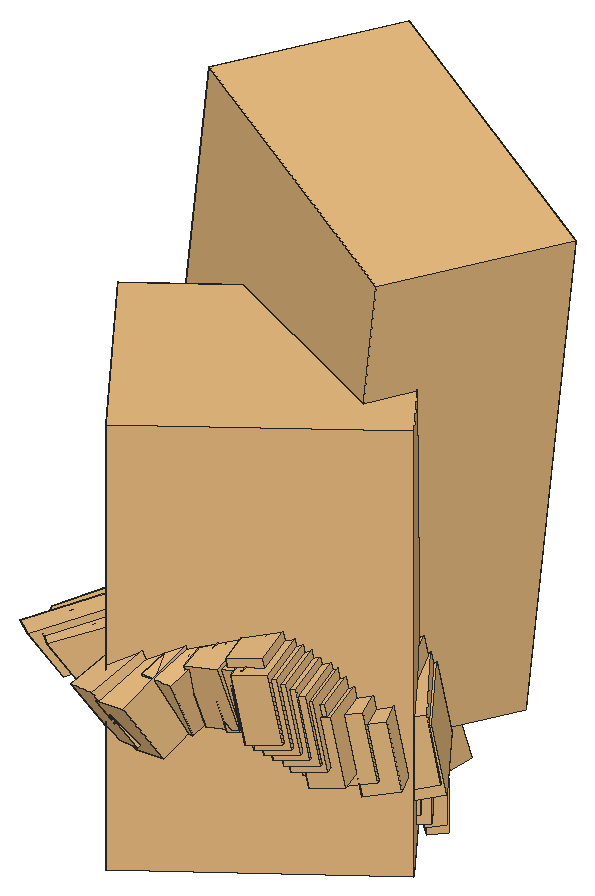
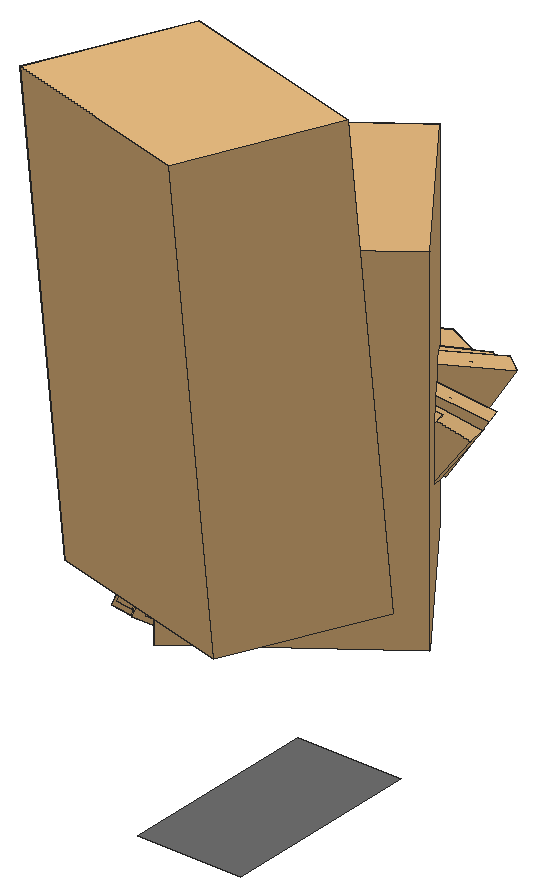
# SketchUp Ruby script. Lengths in inches.
U = 1.inch
M = Sketchup.active_model
def pt(a) = Geom::Point3d.new(a.map { |v| v * U })
def face(e, loops, mat)
  f = e.add_face(loops[0].map { |a| pt(a) })
  loops[1..].each { |l| e.add_face(l.map { |a| pt(a) }).erase! }
  f.material = f.back_material = mat if mat
  f
end
# faces: each face lists its corners as indices into pts; further lists are holes
def faces(e, pts, list, mat = nil) = list.each { |f| face(e, (f[0].is_a?(Array) ? f : [f]).map { |l| l.map { |i| pts[i] } }, mat) }
# xy, xz, yz: faces in a plane at the given z, y or x. An outline is a flat list of corners, or four numbers for a rectangle; further outlines are holes
def ring(l) = l.size == 4 ? [[l[0], l[1]], [l[2], l[1]], [l[2], l[3]], [l[0], l[3]]] : l.each_slice(2).to_a
def flat(e, list, mat, &to3) = list.each { |f| face(e, (f[0].is_a?(Array) ? f : [f]).map { |l| ring(l).map { |u, v| to3.(u, v) } }, mat) }
def xy(e, z, list, mat = nil) = flat(e, list, mat) { |x, y| [x, y, z] }
def xz(e, y, list, mat = nil) = flat(e, list, mat) { |x, z| [x, y, z] }
def yz(e, x, list, mat = nil) = flat(e, list, mat) { |y, z| [x, y, z] }
def lines(e, pts, list) = list.each { |a, b| e.add_line(pt(pts[a]), pt(pts[b])) }
# prism: a flat outline (further loops are holes) pulled along v
def prism(e, loops, v, mat = nil)
  f = face(e, loops, mat); d = Geom::Vector3d.new(v.map { |x| x * U })
  f.pushpull(f.normal.samedirection?(d) ? d.length : -d.length)
end
def box(e, o, s, mat = nil) = prism(e, [[o, [o[0] + s[0], o[1], o[2]], [o[0] + s[0], o[1] + s[1], o[2]], [o[0], o[1] + s[1], o[2]]]], [0, 0, s[2]], mat)
def at(x, y, z, deg = 0) = Geom::Transformation.translation(pt([x, y, z])) * Geom::Transformation.rotation(ORIGIN, Z_AXIS, deg.degrees)
def axes(o, x, y, z) = Geom::Transformation.new([*x, 0, *y, 0, *z, 0, *pt(o).to_a, 1])
def part(name) = M.definitions.add(name)
# library, detail: a bought-in or finely detailed component or shape, given as its bounding box
def library(name, o, s) = part(name).tap { |d| box(d.entities, o, s) }
def detail(e, o, s) = box(e.add_group.entities, o, s)
def put(e, d, t, mat = nil) = e.add_instance(d, t).tap { |i| i.material = mat if mat }
def group(e, t, mat = nil) = e.add_group.tap { |g| g.transformation = t; g.material = mat if mat }.entities
root = M.entities
M.materials.add("AM85_043_stem").color = [137, 75, 57]
M.materials.add("Generic\#4").color = [113, 113, 113]
c1 = library("Group\#263",[26.16,5.88,-22.96],[170.57,196.24,312.95])
c2 = part("Leaf blade")
p = [[83.87,1.9,45.32],[93.74,4.15,37.73],[37.05,-3.5625,61.7],[49.38,-2.58,60.05],[69.4,9.27,54.68],[74.7,9.96,52.16],
  [102.49,6.87,29.18],[110.02,10.09,19.93],[45.83,5.6,61.35],[51.45,6.53,60.35],[91.18,12.19,41.53],[94.56,12.64,38.66],
  [12.82,-5.2,59.53],[24.77,-4.41,61.53],[22.59,0.63,61.46],[34.04,3.3,62.19],[61.47,-1.4,56.68],[73.04,0.08,51.71],
  [109.02,14.97,22.84],[115.89,16.47,11.9375]]
lines(c2.entities,p,[[0,1],[2,3],[4,5],[6,7],[8,9],[10,11],[12,13],[14,15],[16,17],[18,19]])
detail(c2.entities,[1.52,-6.02,0.37],[119.64,24.16,61.82])
c3 = part("Group\#250")
p = [[69.397,177.044,-76.908],[69.056,177.22,-76.772],[69.397,177.397,-76.635],[69.739,177.22,-76.772],[69.397,126.923,-36.489],[68.124,127.405,-35.832],
  [69.397,153.661,-55.129],[70.671,127.405,-35.832],[68.59,154.026,-54.756],[70.205,154.026,-54.756],[69.397,127.887,-35.175],[69.397,154.392,-54.384],
  [69.397,97.5,-21.509],[67.658,98.015,-20.533],[71.137,98.015,-20.533],[69.397,98.53,-19.558],[69.397,66.147,-10.6],[67.192,66.605,-9.289],
  [71.603,66.605,-9.289],[69.397,67.064,-7.977],[69.397,33.682,-4.048],[66.726,33.994,-2.4],[72.069,33.994,-2.4],[69.397,34.304,-0.752],
  [69.397,0.958,-2],[66.26,1.035,-0.035],[69.397,1.112,1.931],[72.535,1.035,-0.035],[69.397,0.956,-2]]
faces(c3.entities,p,[[0,1,2,3]])
faces(c3.entities,p,[[4,5,6],[4,6,7],[8,6,5],[9,7,6],[5,10,11,8],[7,9,11,10],[12,13,4],[12,4,14],
  [5,4,13],[7,14,4],[13,15,10,5],[14,7,10,15],[16,17,12],[16,12,18],[13,12,17],[14,18,12],
  [17,19,15,13],[18,14,15,19],[16,20,17],[16,18,20],[21,17,20],[22,20,18],[21,23,17],[22,18,23],
  [19,17,23],[19,23,18],[20,24,21],[20,22,24],[25,21,24],[25,26,21],[27,24,22],[22,23,27],
  [23,21,26],[28,25,24],[28,27,25],[28,24,27],[26,27,23],[26,25,27]],"AM85_043_stem")
c4 = library("Group\#270",[27.32,5.88,-22.96],[171.91,196.24,312.95])
xy(root,62.5,[[443.58,67.75,455.52,90.9375]],"Generic\#4")
put(root,c1,axes([470.25,54.41,79.57],[0.04473,0.09619,-0.00136],[-0.14118,0.06602,0.02589],[0.02371,-0.00888,0.15193]))
g1 = group(root,at(474.43,72.34,71.32))
put(g1,c2,axes([-12.11,-1.61,3.27],[0.03868,-0.0392,0.03775],[-0.05285,-0.06013,-0.01977],[-0.04833,0.01698,0.0709]))
put(g1,c2,axes([-11.96,-0.56,4.01],[0.04263,-0.04823,0.03034],[-0.05668,-0.05579,-0.02374],[-0.0425,0.00994,0.07598]))
put(g1,c2,axes([-9.03,-15.24,6.15],[0.03132,0.06406,0.00852],[-0.06704,0.0181,-0.03972],[-0.0425,0.00994,0.07598]))
put(g1,c2,axes([-0.71,-1.03,-0.15],[0.01778,-0.047,0.01638],[-0.07034,-0.03079,-0.03479],[-0.0425,0.00994,0.07598]))
put(g1,c2,axes([-18.94,-8.86,3.45],[0.06742,0.02078,0.03933],[0.01295,-0.07484,0.01772],[-0.04843,0.00252,0.04485]))
put(g1,c2,axes([-7.92,0.23,1.4375],[0.0479,-0.05419,0.03409],[-0.05668,-0.05579,-0.02374],[-0.0425,0.00994,0.07598]))
put(g1,c2,axes([-4.09,0.28,0.43],[0.03378,-0.05538,0.02642],[-0.06587,-0.03995,-0.03103],[-0.0425,0.00994,0.07598]))
put(g1,c2,axes([-1.25,-0.99,0.48],[0.01778,-0.047,0.01638],[-0.07034,-0.03079,-0.03479],[-0.0425,0.00994,0.07598]))
put(g1,c2,axes([-7.45,0.48,0.7],[0.0479,-0.05419,0.03409],[-0.05668,-0.05579,-0.02374],[-0.0425,0.00994,0.07598]))
put(g1,c2,axes([-10.4,-14,5.8125],[0.02588,0.05213,0.018],[-0.0646,0.02369,-0.03789],[-0.04616,0.00147,0.07425]))
put(g1,c2,axes([-12.98,-2.44,3.14],[0.0395,-0.03313,0.03981],[-0.04826,-0.06412,-0.01628],[-0.05052,0.01802,0.06901]))
put(g1,c2,axes([-8.82,0.5,1.72],[0.0479,-0.05419,0.03409],[-0.05668,-0.05579,-0.02374],[-0.0425,0.00994,0.07598]))
put(g1,c2,axes([-15.65,-13.52,2.6],[0.04629,0.04424,0.05183],[-0.03259,0.05072,-0.03419],[-0.06385,0.00038,0.05972]))
put(g1,c2,axes([-14.34,-14.04,2.61],[0.03849,0.04933,0.05152],[-0.04598,0.04493,-0.0315],[-0.06071,-0.00886,0.06145]))
put(g1,c2,axes([-6.64,-15.3,5],[0.03132,0.06406,0.00852],[-0.06704,0.0181,-0.03972],[-0.0425,0.00994,0.07598]))
put(g1,c2,axes([-6.11,-15.16,5.27],[0.03132,0.06406,0.00852],[-0.06704,0.0181,-0.03972],[-0.0425,0.00994,0.07598]))
put(g1,c2,axes([-7.43,-15.45,5.63],[0.03132,0.06406,0.00852],[-0.06704,0.0181,-0.03972],[-0.0425,0.00994,0.07598]))
put(g1,c2,axes([-9.33,0.5,2.05],[0.0479,-0.05419,0.03409],[-0.05668,-0.05579,-0.02374],[-0.0425,0.00994,0.07598]))
put(g1,c2,axes([-15.7,-4.11,0.6],[0.04795,-0.01809,0.0661],[-0.02929,-0.07414,-0.00575],[-0.06447,0.01799,0.05565]))
put(g1,c2,axes([-18.72,-10.18,4.28],[0.06811,0.01591,0.04038],[-0.00659,0.06451,-0.01242],[-0.04843,0.00252,0.04485]))
put(g1,c2,axes([-2.05,-14.43,3.48],[0.0178,0.05862,0.00176],[-0.07169,0.00154,-0.04001],[-0.0425,0.00994,0.07598]))
put(g1,c2,axes([0.37,-12.77,2.89],[0.00491,0.04484,-0.00348],[-0.07359,-0.00764,-0.03979],[-0.0425,0.00994,0.07598]))
put(g1,c2,axes([-5.26,-15.32,3.98],[0.03132,0.06406,0.00852],[-0.06704,0.0181,-0.03972],[-0.0425,0.00994,0.07598]))
put(g1,c2,axes([-9.62,-14.86,6.93],[0.02788,0.05702,0.00758],[-0.06704,0.0181,-0.03972],[-0.0425,0.00994,0.07598]))
put(g1,c2,axes([-8.5,-15.29,5.87],[0.03132,0.06406,0.00852],[-0.06704,0.0181,-0.03972],[-0.0425,0.00994,0.07598]))
put(g1,c2,axes([-10.56,0.27,2.66],[0.0479,-0.05419,0.03409],[-0.05668,-0.05579,-0.02374],[-0.0425,0.00994,0.07598]))
put(g1,c2,axes([-11.77,0.21,3.21],[0.0479,-0.05419,0.03409],[-0.05668,-0.05579,-0.02374],[-0.0425,0.00994,0.07598]))
put(g1,c2,axes([-16.81,-5.04,0.9],[0.05394,-0.01033,0.06364],[-0.01462,-0.07744,-0.00647],[-0.06473,0.00665,0.05837]))
put(g1,c2,axes([-11.17,0.24,2.9375],[0.0479,-0.05419,0.03409],[-0.05668,-0.05579,-0.02374],[-0.0425,0.00994,0.07598]))
put(g1,c2,axes([-9.95,0.3,2.38],[0.0479,-0.05419,0.03409],[-0.05668,-0.05579,-0.02374],[-0.0425,0.00994,0.07598]))
put(g1,c2,axes([-9.77,-14.44,6.8],[0.02788,0.05702,0.00758],[-0.06704,0.0181,-0.03972],[-0.0425,0.00994,0.07598]))
put(g1,c2,axes([-14.52,-4.3,2.14],[0.04432,-0.01726,0.05016],[-0.04066,-0.06954,0.00497],[-0.053,0.02967,0.06181]))
put(g1,c2,axes([-11.4375,-13.65,5.43],[0.02804,0.04864,0.02213],[-0.06132,0.02903,-0.03642],[-0.04792,-0.00053,0.07303]))
put(g1,c2,axes([-5.5,0.05,0.88],[0.03829,-0.05246,0.02852],[-0.06335,-0.04371,-0.02912],[-0.0425,0.00994,0.07598]))
put(g1,c2,axes([-8.12,-15.34,6.33],[0.03132,0.06406,0.00852],[-0.06704,0.0181,-0.03972],[-0.0425,0.00994,0.07598]))
put(g1,c2,axes([-13.32,-13.04,3.89],[0.03602,0.042,0.03735],[-0.05638,0.04265,-0.0193],[-0.04711,-0.0123,0.07089]))
put(g1,c2,axes([-3.5,-14.44,3.88],[0.02275,0.05837,0.00455],[-0.07027,0.00563,-0.03979],[-0.0425,0.00994,0.07598]))
put(g1,c3,axes([-0.41,-1.05,-0.14],[0.01308,-0.09333,0.02018],[-0.04855,0.00674,0.06494],[0.06476,0.01996,0.05057]))
put(root,c4,axes([484.52,51.8,73.52],[-0.0818,0.11119,0],[-0.10263,-0.0755,0],[0,0,0.13246]))
g2 = group(root,at(483.76,57.21,77.5))
put(g2,c2,axes([-10.8,-12.78,7.47],[-0.02264,0.10412,0.02015],[-0.12805,-0.034,-0.02131],[-0.01036,-0.02806,0.10296]))
put(g2,c2,axes([-9.16,-12.92,8.5625],[-0.03268,0.11123,0.0078],[-0.12516,-0.04482,-0.02345],[-0.01541,-0.01189,0.10498]))
put(g2,c2,axes([-27.48,3.51,6.11],[0.1159,-0.00379,0.01659],[-0.0298,-0.12528,-0.01857],[-0.01541,-0.01189,0.10498]))
put(g2,c2,axes([-1.14,-0.96,-0.17],[-0.05144,0.0695,0.00032],[-0.10127,-0.08867,-0.02491],[-0.01541,-0.01189,0.10498]))
put(g2,c2,axes([-26.47,-15.79,8.02],[0.08506,0.09563,0.02847],[-0.09456,0.08562,-0.004],[-0.03235,-0.03415,0.06892]))
put(g2,c2,axes([-4.99,-10.07,4.4375],[-0.03672,0.12498,0.00877],[-0.12516,-0.04482,-0.02345],[-0.01541,-0.01189,0.10498]))
put(g2,c2,axes([-1.92,-5.89,1.99],[-0.05004,0.10288,0.00431],[-0.11046,-0.07348,-0.02454],[-0.01541,-0.01189,0.10498]))
put(g2,c2,axes([-1.47,-1.27,0.75],[-0.05144,0.0695,0.00032],[-0.10127,-0.08867,-0.02491],[-0.01541,-0.01189,0.10498]))
put(g2,c2,axes([-4.29,-10.15,3.49],[-0.03672,0.12498,0.00877],[-0.12516,-0.04482,-0.02345],[-0.01541,-0.01189,0.10498]))
put(g2,c2,axes([-26.82,0.58,6.51],[0.09524,0.00467,0.02619],[-0.01986,-0.12528,-0.01577],[-0.03037,-0.01117,0.10193]))
put(g2,c2,axes([-12.68,-13.33,7.39],[-0.01329,0.10185,0.02389],[-0.12985,-0.0228,-0.01989],[-0.01073,-0.03289,0.10179]))
put(g2,c2,axes([-5.3,-11.24,5.14],[-0.03672,0.12498,0.00877],[-0.12516,-0.04482,-0.02345],[-0.01541,-0.01189,0.10498]))
put(g2,c2,axes([-30.49,-8.58,4.68],[0.10217,0.05891,0.05638],[0.04397,-0.10288,-0.01497],[-0.04676,-0.04238,0.09076]))
put(g2,c2,axes([-30.1875,-6.49,4.11],[0.10316,0.04486,0.06],[0.0253,-0.11371,-0.00891],[-0.05724,-0.03015,0.08922]))
put(g2,c2,axes([-25.72,5.84,3.95],[0.1159,-0.00379,0.01659],[-0.0298,-0.12528,-0.01857],[-0.01541,-0.01189,0.10498]))
put(g2,c2,axes([-25.1,6.58,4.125],[0.1159,-0.00379,0.01659],[-0.0298,-0.12528,-0.01857],[-0.01541,-0.01189,0.10498]))
put(g2,c2,axes([-26.53,5.36,4.9],[0.1159,-0.00379,0.01659],[-0.0298,-0.12528,-0.01857],[-0.01541,-0.01189,0.10498]))
put(g2,c2,axes([-5.69,-11.67,5.69],[-0.03672,0.12498,0.00877],[-0.12516,-0.04482,-0.02345],[-0.01541,-0.01189,0.10498]))
put(g2,c2,axes([-17.33,-17.1875,4.92],[0.01615,0.11827,0.05555],[-0.12838,0.01595,-0.01678],[-0.02259,-0.05938,0.09099]))
put(g2,c2,axes([-29.41,-15.15,8.23],[0.07878,0.10093,0.02814],[0.0853,-0.06612,0.00521],[-0.03235,-0.03415,0.06892]))
put(g2,c2,axes([-20.95,10.01,0.88],[0.09709,-0.02125,0.01185],[-0.05691,-0.11866,-0.0218],[-0.01541,-0.01189,0.10498]))
put(g2,c2,axes([-16.71,11.43,-0.17],[0.06709,-0.0305,0.00639],[-0.0714,-0.11387,-0.02338],[-0.01541,-0.01189,0.10498]))
put(g2,c2,axes([-24.71,6.93,2.3],[0.1159,-0.00379,0.01659],[-0.0298,-0.12528,-0.01857],[-0.01541,-0.01189,0.10498]))
put(g2,c2,axes([-27.36,2.97,7.3125],[0.10315,-0.00337,0.01476],[-0.0298,-0.12528,-0.01857],[-0.01541,-0.01189,0.10498]))
put(g2,c2,axes([-27.14,4.04,5.58],[0.1159,-0.00379,0.01659],[-0.0298,-0.12528,-0.01857],[-0.01541,-0.01189,0.10498]))
put(g2,c2,axes([-6.95,-12.65,6.75],[-0.03672,0.12498,0.00877],[-0.12516,-0.04482,-0.02345],[-0.01541,-0.01189,0.10498]))
put(g2,c2,axes([-7.96,-13.79,7.79],[-0.03672,0.12498,0.00877],[-0.12516,-0.04482,-0.02345],[-0.01541,-0.01189,0.10498]))
put(g2,c2,axes([-19.52,-17.68,5.39],[0.03173,0.11833,0.05277],[-0.12145,0.03667,-0.02344],[-0.03867,-0.04921,0.09118]))
put(g2,c2,axes([-7.46,-13.23,7.27],[-0.03672,0.12498,0.00877],[-0.12516,-0.04482,-0.02345],[-0.01541,-0.01189,0.10498]))
put(g2,c2,axes([-6.44,-12.09,6.23],[-0.03672,0.12498,0.00877],[-0.12516,-0.04482,-0.02345],[-0.01541,-0.01189,0.10498]))
put(g2,c2,axes([-26.89,2.375,7.3125],[0.10315,-0.00337,0.01476],[-0.0298,-0.12528,-0.01857],[-0.01541,-0.01189,0.10498]))
put(g2,c2,axes([-16.58,-14.52,6.25],[0.01355,0.10258,0.03854],[-0.13029,0.00497,0.0007],[0.00337,-0.04971,0.09742]))
put(g2,c2,axes([-27.18,-1.25,6.51],[0.09225,0.01281,0.0293],[-0.00962,-0.12424,-0.01373],[-0.03467,-0.01269,0.10057]))
put(g2,c2,axes([-3.35,-7.21,2.93],[-0.04221,0.10776,0.00601],[-0.11368,-0.06612,-0.02418],[-0.01541,-0.01189,0.10498]))
put(g2,c2,axes([-26.89,4.86,5.98],[0.1159,-0.00379,0.01659],[-0.0298,-0.12528,-0.01857],[-0.01541,-0.01189,0.10498]))
put(g2,c2,axes([-27.9,-5.13,5.53],[0.09003,0.03805,0.04245],[0.0145,-0.11719,0.00811],[-0.0508,-0.00401,0.09465]))
put(g2,c2,axes([-22.09,8.44,1.83],[0.10083,-0.01292,0.01334],[-0.05,-0.11985,-0.02092],[-0.01541,-0.01189,0.10498]))
put(g2,c3,axes([-0.92,-0.57,-0.26],[-0.12045,0.10163,-0.00617],[-0.02534,-0.02437,0.09337],[0.08241,0.10024,0.04215]))
g3 = group(root,at(480.63,61.3,70.7))
put(g3,c2,axes([-4.45,-7.11,7.62],[-0.0221,0.05477,0.00846],[-0.06568,-0.0337,0.00097],[0.00432,-0.00825,0.07805]))
put(g3,c2,axes([-3.49,-6.92,8.24],[-0.02902,0.05654,0],[-0.0631,-0.03933,0],[0,0,0.07872]))
put(g3,c2,axes([-15.18,-0.31,7.0625],[0.06305,0.01181,0],[-0.00333,-0.07165,0],[0,0,0.07872]))
put(g3,c2,axes([-1.12,-0.32,0.07],[-0.0349,0.03162,0],[-0.04571,-0.06031,0],[0,0,0.07872]))
put(g3,c2,axes([-12.41,-10.37,9.93],[0.03657,0.06254,0.00373],[-0.05985,0.03523,0.00013],[-0.00892,-0.0165,0.05621]))
put(g3,c2,axes([-1.86,-5.26,4.58],[-0.0326,0.06353,0],[-0.0631,-0.03933,0],[0,0,0.07872]))
put(g3,c2,axes([-0.85,-2.88,2.13],[-0.03755,0.04992,0],[-0.05223,-0.05315,0],[0,0,0.07872]))
put(g3,c2,axes([-1.2,-0.45,0.81],[-0.0349,0.03162,0],[-0.04571,-0.06031,0],[0,0,0.07872]))
put(g3,c2,axes([-1.54,-5.3,3.82],[-0.0326,0.06353,0],[-0.0631,-0.03933,0],[0,0,0.07872]))
put(g3,c2,axes([-14.49,-1.77,7.53],[0.05178,0.01483,0.00846],[0.00212,-0.07036,0.00097],[-0.00822,-0.00147,0.07805]))
put(g3,c2,axes([-5.39,-7.61,7.8],[-0.01664,0.05486,0.01037],[-0.06777,-0.02779,0.00127],[0.00457,-0.01096,0.07764]))
put(g3,c2,axes([-1.85,-5.86,5.21],[-0.0326,0.06353,0],[-0.0631,-0.03933,0],[0,0,0.07872]))
put(g3,c2,axes([-15.55,-7.21,7.35],[0.05151,0.04689,0.02516],[0.03362,-0.0514,-0.00708],[-0.01425,-0.02079,0.07426]))
put(g3,c2,axes([-15.66,-6.1,6.73],[0.05381,0.03977,0.02884],[0.02529,-0.05875,0.00019],[-0.02125,-0.0155,0.07325]))
put(g3,c2,axes([-14.64,0.96,5.12],[0.06305,0.01181,0],[-0.00333,-0.07165,0],[0,0,0.07872]))
put(g3,c2,axes([-14.38,1.44,5.12],[0.06305,0.01181,0],[-0.00333,-0.07165,0],[0,0,0.07872]))
put(g3,c2,axes([-14.96,0.69,5.9375],[0.06305,0.01181,0],[-0.00333,-0.07165,0],[0,0,0.07872]))
put(g3,c2,axes([-1.98,-6.1,5.69],[-0.0326,0.06353,0],[-0.0631,-0.03933,0],[0,0,0.07872]))
put(g3,c2,axes([-7.6,-10.37,6.82],[-0.00072,0.06925,0.02884],[-0.07102,-0.00667,0.00019],[0.00047,-0.02725,0.07325]))
put(g3,c2,axes([-13.44,-9.52,10.34],[0.03264,0.06467,0.00373],[0.05288,-0.02571,0.00013],[-0.00892,-0.0165,0.05621]))
put(g3,c2,axes([-12.77,3.47,2.04],[0.05466,0.00007,0],[-0.01867,-0.0713,0],[0,0,0.07872]))
put(g3,c2,axes([-10.74,4.62,0.72],[0.03939,-0.00855,0],[-0.02699,-0.07043,0],[0,0,0.07872]))
put(g3,c2,axes([-14.34,1.53,3.73],[0.06305,0.01181,0],[-0.00333,-0.07165,0],[0,0,0.07872]))
put(g3,c2,axes([-14.98,-0.49,7.97],[0.05611,0.01051,0],[-0.00333,-0.07165,0],[0,0,0.07872]))
put(g3,c2,axes([-15.09,-0.03,6.61],[0.06305,0.01181,0],[-0.00333,-0.07165,0],[0,0,0.07872]))
put(g3,c2,axes([-2.47,-6.68,6.67],[-0.0326,0.06353,0],[-0.0631,-0.03933,0],[0,0,0.07872]))
put(g3,c2,axes([-2.8125,-7.3125,7.625],[-0.0326,0.06353,0],[-0.0631,-0.03933,0],[0,0,0.07872]))
put(g3,c2,axes([-8.68,-10.83,7.4375],[0.00736,0.07076,0.02516],[-0.07005,0.00465,-0.00708],[-0.00917,-0.02353,0.07426]))
put(g3,c2,axes([-2.64,-7,7.15],[-0.0326,0.06353,0],[-0.0631,-0.03933,0],[0,0,0.07872]))
put(g3,c2,axes([-2.3,-6.36,6.2],[-0.0326,0.06353,0],[-0.0631,-0.03933,0],[0,0,0.07872]))
put(g3,c2,axes([-14.67,-0.76,7.97],[0.05611,0.01051,0],[-0.00333,-0.07165,0],[0,0,0.07872]))
put(g3,c2,axes([-7.41,-8.76,7.49],[-0.0015,0.05927,0.01807],[-0.06969,-0.01142,0.01396],[0.01362,-0.01877,0.07435]))
put(g3,c2,axes([-14.48,-2.79,7.71],[0.04951,0.01909,0.01037],[0.00758,-0.06854,0.00127],[-0.01043,-0.00285,0.07764]))
put(g3,c2,axes([-1.4,-3.67,3.08],[-0.03381,0.05351,0],[-0.05472,-0.04954,0],[0,0,0.07872]))
put(g3,c2,axes([-15.02,0.47,6.8],[0.06305,0.01181,0],[-0.00333,-0.07165,0],[0,0,0.07872]))
put(g3,c2,axes([-14.5,-5.02,7.4],[0.04643,0.03336,0.01807],[0.02106,-0.06048,0.01396],[-0.02034,-0.00041,0.07435]))
put(g3,c2,axes([-13.14,2.59,2.98],[0.05583,0.00504,0],[-0.01481,-0.07112,0],[0,0,0.07872]))
put(g3,c3,axes([-1.05,-0.1,-0.04],[-0.07549,0.04082,0],[-0.00467,-0.00864,0.07239],[0.03556,0.06577,0.01355]))
